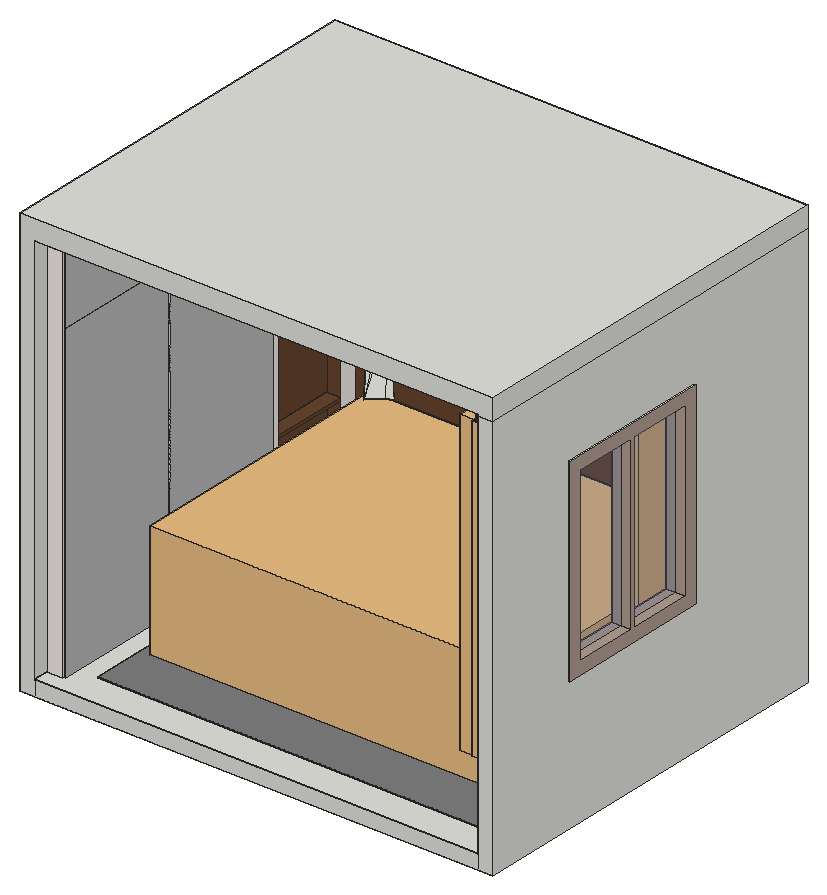
# SketchUp Ruby script. Lengths in inches.
U = 1.inch
M = Sketchup.active_model
def pt(a) = Geom::Point3d.new(a.map { |v| v * U })
def face(e, loops, mat)
  f = e.add_face(loops[0].map { |a| pt(a) })
  loops[1..].each { |l| e.add_face(l.map { |a| pt(a) }).erase! }
  f.material = f.back_material = mat if mat
  f
end
# faces: each face lists its corners as indices into pts; further lists are holes
def faces(e, pts, list, mat = nil) = list.each { |f| face(e, (f[0].is_a?(Array) ? f : [f]).map { |l| l.map { |i| pts[i] } }, mat) }
# xy, xz, yz: faces in a plane at the given z, y or x. An outline is a flat list of corners, or four numbers for a rectangle; further outlines are holes
def ring(l) = l.size == 4 ? [[l[0], l[1]], [l[2], l[1]], [l[2], l[3]], [l[0], l[3]]] : l.each_slice(2).to_a
def flat(e, list, mat, &to3) = list.each { |f| face(e, (f[0].is_a?(Array) ? f : [f]).map { |l| ring(l).map { |u, v| to3.(u, v) } }, mat) }
def xy(e, z, list, mat = nil) = flat(e, list, mat) { |x, y| [x, y, z] }
def xz(e, y, list, mat = nil) = flat(e, list, mat) { |x, z| [x, y, z] }
def yz(e, x, list, mat = nil) = flat(e, list, mat) { |y, z| [x, y, z] }
def lines(e, pts, list) = list.each { |a, b| e.add_line(pt(pts[a]), pt(pts[b])) }
# prism: a flat outline (further loops are holes) pulled along v
def prism(e, loops, v, mat = nil)
  f = face(e, loops, mat); d = Geom::Vector3d.new(v.map { |x| x * U })
  f.pushpull(f.normal.samedirection?(d) ? d.length : -d.length)
end
def box(e, o, s, mat = nil) = prism(e, [[o, [o[0] + s[0], o[1], o[2]], [o[0] + s[0], o[1] + s[1], o[2]], [o[0], o[1] + s[1], o[2]]]], [0, 0, s[2]], mat)
def at(x, y, z, deg = 0) = Geom::Transformation.translation(pt([x, y, z])) * Geom::Transformation.rotation(ORIGIN, Z_AXIS, deg.degrees)
def axes(o, x, y, z) = Geom::Transformation.new([*x, 0, *y, 0, *z, 0, *pt(o).to_a, 1])
def part(name) = M.definitions.add(name)
# library, detail: a bought-in or finely detailed component or shape, given as its bounding box
def library(name, o, s) = part(name).tap { |d| box(d.entities, o, s) }
def detail(e, o, s) = box(e.add_group.entities, o, s)
def put(e, d, t, mat = nil) = e.add_instance(d, t).tap { |i| i.material = mat if mat }
def group(e, t, mat = nil) = e.add_group.tap { |g| g.transformation = t; g.material = mat if mat }.entities
root = M.entities
M.materials.add("0209 AP 9428 SKY PINK").color = [243, 236, 233]
M.materials.add("2036 AP 8776 DARK ASH").color = [176, 158, 145]
M.materials.add("DDR840RVS01100X").color = [126, 127, 125]
M.materials.add("Glass_Mirror_01").color = [185, 185, 185]
M.materials.add("Glass_Sky Reflection_01").color = [126, 138, 183]
M.materials["Glass_Sky Reflection_01"].alpha = 0.25
M.materials.add("Wood_Veneer_15_1K").color = [103, 69, 45]
c1 = library("Double bed",[0,0,0],[83.59,112.46,35.43])
c2 = part("Carpet v15 (4)")
xy(c2.entities,0,[[-70.87,0,47.24,78.74]])
xy(c2.entities,0.39,[[-70.87,0,47.24,78.74]],"DDR840RVS01100X")
xz(c2.entities,0,[[-70.87,0,47.24,0.39]])
xz(c2.entities,78.74,[[-70.87,0,47.24,0.39]])
yz(c2.entities,-70.87,[[0,0,78.74,0.39]])
yz(c2.entities,47.24,[[0,0,78.74,0.39]])
c3 = part("Group\#8")
g1 = group(c3.entities,at(1.62,23.48,0.37))
prism(g1,[[[2.19,-1.21,0],[0.78,-1.47,0],[-0.07,3.1,0],[1.34,3.36,0]]],[0,0,0.04])
g2 = group(c3.entities,at(0,0,0))
xy(g2,0.33,[[3.33,0,0,23.09,1.89,23.4375],[3.33,0,1.89,23.4375,2.83,23.62],[3.33,0,2.83,23.62,4.25,23.88,8.53,0.97,7.12,0.71]])
xy(g2,0.37,[[3.33,0,1.89,23.4375,0,23.09],[3.33,0,2.83,23.62,1.89,23.4375],[3.33,0,7.12,0.71,8.53,0.97,4.25,23.88,2.83,23.62]])
p = [[5.64,24.14,0.12],[4.25,23.88,0.37],[8.53,0.97,0.37],[10.39,1.32,0.04],[4.25,23.88,0.33],[5.64,24.14,0.08],
  [10.39,1.32,0],[8.53,0.97,0.33],[2.83,23.62,0.33],[1.89,23.4375,0.33],[0,23.09,0.33],[0,23.09,0.37],
  [1.89,23.4375,0.37],[2.83,23.62,0.37],[3.33,0,0.33],[3.33,0,0.37],[7.12,0.71,0.37],[7.12,0.71,0.33]]
faces(g2,p,[[0,1,2,3],[4,5,6,7],[6,3,2,7],[5,0,3,6],[0,5,4,8,9,10,11,12,13,1],[14,15,11,10],[7,2,16,15,14,17]])
c4 = part("ceiling fan")
g3 = group(c4.entities,at(0.63,30.3,-2.8,-91.2))
g4 = group(g3,at(24.19,24.96,0))
xy(g4,0,[[4.53,2.58,4.03,2.65,3.56,2.84,3.16,3.15,2.85,3.55,2.65,4.02,2.58,4.52,2.65,5.02,2.84,5.5,3.15,5.9,3.55,6.21,4.02,6.41,4.52,6.47,5.02,6.41,5.5,6.22,5.9,5.91,6.21,5.51,6.41,5.04,6.47,4.53,6.41,4.03,6.22,3.56,5.91,3.16,5.51,2.85,5.04,2.65]])
xy(g4,2.76,[[4.54,0,5.71,0.16,6.8,0.61,7.74,1.34,8.46,2.28,8.9,3.37,9.06,4.54,8.9,5.71,8.44,6.8,7.72,7.74,6.78,8.46,5.68,8.9,4.51,9.06,3.34,8.9,2.25,8.44,1.32,7.72,0.6,6.78,0.15,5.68,0,4.51,0.16,3.34,0.61,2.25,1.34,1.32,2.28,0.6,3.37,0.15]])
p = [[4.54,0,1.57],[3.37,0.15,1.57],[4.03,2.65,0],[4.53,2.58,0],[5.71,0.16,1.57],[5.04,2.65,0],
  [2.28,0.6,1.57],[3.56,2.84,0],[6.8,0.61,1.57],[5.51,2.85,0],[1.34,1.32,1.57],[3.16,3.15,0],
  [7.74,1.34,1.57],[5.91,3.16,0],[0.61,2.25,1.57],[2.85,3.55,0],[8.46,2.28,1.57],[6.22,3.56,0],
  [0.16,3.34,1.57],[2.65,4.02,0],[8.9,3.37,1.57],[6.41,4.03,0],[0,4.51,1.57],[2.58,4.52,0],
  [9.06,4.54,1.57],[6.47,4.53,0],[0.15,5.68,1.57],[2.65,5.02,0],[8.9,5.71,1.57],[6.41,5.04,0],
  [0.6,6.78,1.57],[2.84,5.5,0],[8.44,6.8,1.57],[6.21,5.51,0],[1.32,7.72,1.57],[3.15,5.9,0],
  [7.72,7.74,1.57],[5.9,5.91,0],[2.25,8.44,1.57],[3.55,6.21,0],[6.78,8.46,1.57],[5.5,6.22,0],
  [3.34,8.9,1.57],[4.02,6.41,0],[5.68,8.9,1.57],[5.02,6.41,0],[4.51,9.06,1.57],[4.52,6.47,0],
  [3.37,0.15,2.76],[4.54,0,2.76],[5.71,0.16,2.76],[2.28,0.6,2.76],[6.8,0.61,2.76],[1.34,1.32,2.76],
  [7.74,1.34,2.76],[0.61,2.25,2.76],[8.46,2.28,2.76],[0.16,3.34,2.76],[8.9,3.37,2.76],[0,4.51,2.76],
  [9.06,4.54,2.76],[0.15,5.68,2.76],[8.9,5.71,2.76],[0.6,6.78,2.76],[8.44,6.8,2.76],[1.32,7.72,2.76],
  [7.72,7.74,2.76],[2.25,8.44,2.76],[6.78,8.46,2.76],[3.34,8.9,2.76],[5.68,8.9,2.76],[4.51,9.06,2.76]]
faces(g4,p,[[0,1,2,3],[4,0,3,5],[1,6,7,2],[8,4,5,9],[6,10,11,7],[12,8,9,13],[10,14,15,11],[16,12,13,17],
  [14,18,19,15],[20,16,17,21],[18,22,23,19],[24,20,21,25],[22,26,27,23],[28,24,25,29],[26,30,31,27],[32,28,29,33],
  [30,34,35,31],[36,32,33,37],[34,38,39,35],[40,36,37,41],[38,42,43,39],[44,40,41,45],[42,46,47,43],[46,44,45,47],
  [48,1,0,49],[49,0,4,50],[51,6,1,48],[50,4,8,52],[53,10,6,51],[52,8,12,54],[55,14,10,53],[54,12,16,56],
  [57,18,14,55],[56,16,20,58],[59,22,18,57],[58,20,24,60],[61,26,22,59],[60,24,28,62],[63,30,26,61],[62,28,32,64],
  [65,34,30,63],[64,32,36,66],[67,38,34,65],[66,36,40,68],[69,42,38,67],[68,40,44,70],[71,46,42,69],[70,44,46,71]])
put(g3,c3,at(26.98,0,2.42))
put(g3,c3,at(4.05,45.73,2.42,-120))
put(g3,c3,at(55.12,42.72,2.42,120))
g5 = group(g3,at(25.76,26.53,17.72))
p = [[2.95,2.95,7.28],[2.95,2.95,5.91]]
lines(g5,p,[[0,1]])
g6 = group(g5,at(0,0,5.91))
xy(g6,-5.91,[[[2.95,1.99,2.7,2.02,2.47,2.12,2.27,2.27,2.12,2.47,2.02,2.7,1.99,2.95,2.02,3.2,2.12,3.4375,2.27,3.64,2.47,3.79,2.7,3.89,2.95,3.92,3.2,3.89,3.4375,3.79,3.64,3.64,3.79,3.4375,3.89,3.2,3.92,2.95,3.89,2.7,3.79,2.47,3.64,2.27,3.4375,2.12,3.2,2.02],[2.95,2.38,3.1,2.4,3.24,2.46,3.36,2.55,3.45,2.67,3.5,2.81,3.52,2.95,3.5,3.1,3.45,3.24,3.36,3.36,3.24,3.45,3.1,3.5,2.95,3.52,2.81,3.5,2.67,3.45,2.55,3.36,2.46,3.24,2.4,3.1,2.38,2.95,2.4,2.81,2.46,2.67,2.55,2.55,2.67,2.46,2.81,2.4]]])
xy(g6,0,[[2.95,0,3.72,0.1,4.43,0.4,5.04,0.86,5.51,1.48,5.8,2.1875,5.91,2.95,5.8,3.72,5.51,4.43,5.04,5.04,4.43,5.51,3.72,5.8,2.95,5.91,2.1875,5.8,1.48,5.51,0.86,5.04,0.4,4.43,0.1,3.72,0,2.95,0.1,2.1875,0.4,1.48,0.86,0.86,1.48,0.4,2.1875,0.1]])
p = [[2.95,0,0],[2.1875,0.1,0],[2.7,2.02,-5.91],[2.95,1.99,-5.91],[3.72,0.1,0],[3.2,2.02,-5.91],
  [1.48,0.4,0],[2.47,2.12,-5.91],[4.43,0.4,0],[3.4375,2.12,-5.91],[0.86,0.86,0],[2.27,2.27,-5.91],
  [5.04,0.86,0],[3.64,2.27,-5.91],[0.4,1.48,0],[2.12,2.47,-5.91],[5.51,1.48,0],[3.79,2.47,-5.91],
  [0.1,2.1875,0],[2.02,2.7,-5.91],[5.8,2.1875,0],[3.89,2.7,-5.91],[0,2.95,0],[1.99,2.95,-5.91],
  [5.91,2.95,0],[3.92,2.95,-5.91],[0.1,3.72,0],[2.02,3.2,-5.91],[5.8,3.72,0],[3.89,3.2,-5.91],
  [0.4,4.43,0],[2.12,3.4375,-5.91],[5.51,4.43,0],[3.79,3.4375,-5.91],[0.86,5.04,0],[2.27,3.64,-5.91],
  [5.04,5.04,0],[3.64,3.64,-5.91],[1.48,5.51,0],[2.47,3.79,-5.91],[4.43,5.51,0],[3.4375,3.79,-5.91],
  [2.1875,5.8,0],[2.7,3.89,-5.91],[3.72,5.8,0],[3.2,3.89,-5.91],[2.95,5.91,0],[2.95,3.92,-5.91]]
faces(g6,p,[[0,1,2,3],[4,0,3,5],[1,6,7,2],[8,4,5,9],[6,10,11,7],[12,8,9,13],[10,14,15,11],[16,12,13,17],
  [14,18,19,15],[20,16,17,21],[18,22,23,19],[24,20,21,25],[22,26,27,23],[28,24,25,29],[26,30,31,27],[32,28,29,33],
  [30,34,35,31],[36,32,33,37],[34,38,39,35],[40,36,37,41],[38,42,43,39],[44,40,41,45],[42,46,47,43],[46,44,45,47]])
g7 = group(g3,at(25.76,26.53,1.46))
xy(g7,0,[[2.95,0,3.72,0.1,4.43,0.4,5.04,0.86,5.51,1.48,5.8,2.1875,5.91,2.95,5.8,3.72,5.51,4.43,5.04,5.04,4.43,5.51,3.72,5.8,2.95,5.91,2.1875,5.8,1.48,5.51,0.86,5.04,0.4,4.43,0.1,3.72,0,2.95,0.1,2.1875,0.4,1.48,0.86,0.86,1.48,0.4,2.1875,0.1]])
xy(g7,5.91,[[[2.95,1.99,2.7,2.02,2.47,2.12,2.27,2.27,2.12,2.47,2.02,2.7,1.99,2.95,2.02,3.2,2.12,3.4375,2.27,3.64,2.47,3.79,2.7,3.89,2.95,3.92,3.2,3.89,3.4375,3.79,3.64,3.64,3.79,3.4375,3.89,3.2,3.92,2.95,3.89,2.7,3.79,2.47,3.64,2.27,3.4375,2.12,3.2,2.02],[2.95,2.38,3.1,2.4,3.24,2.46,3.36,2.55,3.45,2.67,3.5,2.81,3.52,2.95,3.5,3.1,3.45,3.24,3.36,3.36,3.24,3.45,3.1,3.5,2.95,3.52,2.81,3.5,2.67,3.45,2.55,3.36,2.46,3.24,2.4,3.1,2.38,2.95,2.4,2.81,2.46,2.67,2.55,2.55,2.67,2.46,2.81,2.4]]])
p = [[2.95,0,0],[2.1875,0.1,0],[2.7,2.02,5.91],[2.95,1.99,5.91],[3.72,0.1,0],[3.2,2.02,5.91],
  [1.48,0.4,0],[2.47,2.12,5.91],[4.43,0.4,0],[3.4375,2.12,5.91],[0.86,0.86,0],[2.27,2.27,5.91],
  [5.04,0.86,0],[3.64,2.27,5.91],[0.4,1.48,0],[2.12,2.47,5.91],[5.51,1.48,0],[3.79,2.47,5.91],
  [0.1,2.1875,0],[2.02,2.7,5.91],[5.8,2.1875,0],[3.89,2.7,5.91],[0,2.95,0],[1.99,2.95,5.91],
  [5.91,2.95,0],[3.92,2.95,5.91],[0.1,3.72,0],[2.02,3.2,5.91],[5.8,3.72,0],[3.89,3.2,5.91],
  [0.4,4.43,0],[2.12,3.4375,5.91],[5.51,4.43,0],[3.79,3.4375,5.91],[0.86,5.04,0],[2.27,3.64,5.91],
  [5.04,5.04,0],[3.64,3.64,5.91],[1.48,5.51,0],[2.47,3.79,5.91],[4.43,5.51,0],[3.4375,3.79,5.91],
  [2.1875,5.8,0],[2.7,3.89,5.91],[3.72,5.8,0],[3.2,3.89,5.91],[2.95,5.91,0],[2.95,3.92,5.91]]
faces(g7,p,[[0,1,2,3],[4,0,3,5],[1,6,7,2],[8,4,5,9],[6,10,11,7],[12,8,9,13],[10,14,15,11],[16,12,13,17],
  [14,18,19,15],[20,16,17,21],[18,22,23,19],[24,20,21,25],[22,26,27,23],[28,24,25,29],[26,30,31,27],[32,28,29,33],
  [30,34,35,31],[36,32,33,37],[34,38,39,35],[40,36,37,41],[38,42,43,39],[44,40,41,45],[42,46,47,43],[46,44,45,47]])
g8 = group(g3,at(25.76,26.53,27.76))
prism(g8,[[[2.95,2.38,-20.39],[2.81,2.4,-20.39],[2.67,2.46,-20.39],[2.55,2.55,-20.39],[2.46,2.67,-20.39],[2.4,2.81,-20.39],[2.38,2.95,-20.39],[2.4,3.1,-20.39],[2.46,3.24,-20.39],[2.55,3.36,-20.39],[2.67,3.45,-20.39],[2.81,3.5,-20.39],[2.95,3.52,-20.39],[3.1,3.5,-20.39],[3.24,3.45,-20.39],[3.36,3.36,-20.39],[3.45,3.24,-20.39],[3.5,3.1,-20.39],[3.52,2.95,-20.39],[3.5,2.81,-20.39],[3.45,2.67,-20.39],[3.36,2.55,-20.39],[3.24,2.46,-20.39],[3.1,2.4,-20.39]]],[0,0,10.35])
c5 = part("Group28\#2")
xy(c5.entities,0,[[-20.0625,-26.0625,-0.59,26.0625],[0.59,-26.0625,20.0625,26.0625]])
c6 = library("Group16",[86.37,-10.76,76.46],[21.79,14.87,35.97])
c7 = library("Group22",[48.82,-10.91,0.23],[97.72,18.57,293.12])
c8 = library("Group24",[44.03,2.01,0.26],[103.73,11,292.35])
c9 = library("Group27",[-106.21,-10.76,76.46],[21.8,14.87,35.97])
c10 = library("Group35",[-145.81,2.01,0.26],[103.73,11,292.35])
c11 = library("Group33",[-144.59,-10.91,0.23],[97.72,18.57,293.12])
xy(root,-4.39,[[0,0,144,120]])
xy(root,0,[[4.5,0,139.5,0,139.5,115.5,9.5,115.5,9.5,110.5,5,110.5,5,86.5,9.5,86.5,9.5,4.5,4.5,4.5]])
xy(root,0.39,[[4.5,0,139.5,0,139.5,115.5,139.26,115.5,139.26,114.79,122.85,114.79,122.85,115.5,9.5,115.5,9.5,110.5,5,110.5,5,86.5,9.5,86.5,9.5,4.5,4.5,4.5],[135.32,102.33,139.5,109.79],[122.85,114.79,139.26,115.5]])
xy(root,0.63,[[9.5,4.74,10.21,44.06],[9.5,44.29,10.21,83.62]])
xy(root,29.61,[[5,86.5,9.5,110.5]],"Wood_Veneer_15_1K")
xy(root,30.39,[[5,86.5,9.5,110.5]],"Wood_Veneer_15_1K")
xy(root,36.39,[[139.5,28.5,141.75,76.5],[141.75,28.5,144,76.5],[144,28.5,144.6875,76.5]])
xy(root,36.39,[[138.8125,28.5,139.5,76.5]],"2036 AP 8776 DARK ASH")
xy(root,40.33,[[138.8125,32.4375,144.6875,51.91],[138.8125,53.09,144.6875,72.5625]],"2036 AP 8776 DARK ASH")
xy(root,48,[[122.85,114.79,139.26,115.5]])
xy(root,48.24,[[9.74,114.79,26.86,115.5],[27.1,114.79,45.19,115.5],[45.43,114.79,80.1,115.5],[80.34,114.79,106.69,115.5],[106.93,114.79,122.48,115.5],
  [122.71,114.79,139.26,115.5]])
xy(root,59.58,[[5,86.5,9.5,110.5]],"Wood_Veneer_15_1K")
xy(root,60.39,[[5,86.5,9.5,110.5]],"Wood_Veneer_15_1K")
xy(root,89.61,[[5,86.5,9.5,110.5]],"Wood_Veneer_15_1K")
xy(root,90.39,[[5,86.5,9.5,110.5]])
xy(root,92.46,[[138.8125,32.4375,144.6875,51.91],[138.8125,53.09,144.6875,72.5625]])
xy(root,95.83,[[9.5,4.74,10.21,44.06],[9.5,44.29,10.21,83.62]])
xy(root,96.07,[[9.5,4.74,10.21,44.06],[9.5,44.29,10.21,83.62]])
xy(root,96.39,[[139.5,28.5,141.75,76.5],[141.75,28.5,144,76.5],[144,28.5,144.6875,76.5]])
xy(root,96.39,[[138.8125,28.5,139.5,76.5]],"2036 AP 8776 DARK ASH")
xy(root,114.61,[[135.32,4.5,135.25,109.79,139.43,109.79,139.5,4.5]])
xy(root,119.37,[[9.5,4.74,10.21,44.06],[9.5,44.29,10.21,83.62]])
xy(root,119.61,[[9.74,114.79,26.86,115.5],[27.1,114.79,45.19,115.5],[45.43,114.79,80.1,115.5],[80.34,114.79,106.69,115.5],[106.93,114.79,122.48,115.5],
  [122.71,114.79,139.26,115.5]])
xy(root,120,[[[4.5,0,4.5,4.5,9.5,4.5,9.5,86.5,5,86.5,5,110.5,9.5,110.5,9.5,115.5,139.5,115.5,139.5,0],[25.7,16.2,123.3,99.3]],[135.32,4.5,139.5,4.5,139.43,109.79,135.25,109.79]])
xy(root,121.5,[[22.82,16.2,25.7,99.3],[123.3,16.2,126.18,102.18],[22.82,99.3,123.3,102.18]])
xy(root,123,[[22.82,16.2,126.18,102.18]])
xy(root,126,[[0,0,144,120]])
xz(root,0,[[0,-4.39,4.5,-4.39,4.5,120,139.5,120,139.5,119.61,144,119.61,144,126,0,126],[4.5,-4.39,139.5,0],[139.5,-4.39,144,119.61]])
xz(root,4.5,[[135.32,114.61,139.5,119.61],[4.5,119.61,9.5,120],[135.32,119.61,139.5,120],[4.5,120,9.5,120.39]])
xz(root,4.5,[[4.5,0.39,9.5,119.61]],"0209 AP 9428 SKY PINK")
xz(root,4.74,[[9.5,0.63,10.21,95.83],[9.5,96.07,10.21,119.37]])
xz(root,16.2,[[25.7,120,25.7,121.5,22.82,121.5,22.82,123,126.18,123,126.18,121.5,123.3,121.5,123.3,120]])
xz(root,28.5,[[139.5,36.39,141.75,96.39],[141.75,36.39,144,96.39],[144,36.39,144.6875,96.39]])
xz(root,28.5,[[138.8125,36.39,139.5,96.39]],"2036 AP 8776 DARK ASH")
xz(root,32.4375,[[138.8125,40.33,144.6875,92.46]])
xz(root,44.06,[[9.5,0.63,10.21,95.83],[9.5,96.07,10.21,119.37]])
xz(root,44.29,[[9.5,0.63,10.21,95.83],[9.5,96.07,10.21,119.37]])
xz(root,51.91,[[138.8125,40.33,144.6875,92.46]],"2036 AP 8776 DARK ASH")
xz(root,53.09,[[138.8125,40.33,144.6875,92.46]])
xz(root,72.5625,[[138.8125,40.33,144.6875,92.46]],"2036 AP 8776 DARK ASH")
xz(root,76.5,[[138.8125,36.39,139.5,96.39],[139.5,36.39,141.75,96.39],[141.75,36.39,144,96.39],[144,36.39,144.6875,96.39]])
xz(root,83.62,[[9.5,0.63,10.21,95.83],[9.5,96.07,10.21,119.37]])
xz(root,86.5,[[5,0,9.5,0.39],[5,0.39,9.5,29.61],[5,29.61,9.5,30],[5,30,9.5,30.39],[5,30.39,9.5,59.58],
  [5,60.39,9.5,89.61],[5,90.39,9.5,119.61],[5,119.61,9.5,120],[5,120,9.5,120.39]])
xz(root,99.3,[[25.7,120,123.3,121.5]])
xz(root,102.18,[[22.82,121.5,126.18,123]])
xz(root,102.33,[[135.32,0.39,139.5,0.39,139.43,114.61,135.25,114.6]],"0209 AP 9428 SKY PINK")
xz(root,109.79,[[135.32,0.39,135.25,114.6,139.43,114.61,139.5,0.39],[135.25,114.61,139.43,120]])
xz(root,110.5,[[5,29.61,9.5,30.39],[5,119.61,9.5,120],[5,120,9.5,120.39]])
xz(root,110.5,[[5,0.39,9.5,29.61],[5,30.39,9.5,59.58],[5,60.39,9.5,89.61],[5,90.39,9.5,119.61]],"Wood_Veneer_15_1K")
xz(root,114.79,[[9.74,48.24,26.86,119.61],[27.1,48.24,45.19,119.61],[45.43,48.24,80.1,119.61],[80.34,48.24,106.69,119.61],[106.93,48.24,122.48,119.61],
  [122.71,48.24,139.26,119.61]])
xz(root,114.79,[[122.85,0.39,139.26,48]],"0209 AP 9428 SKY PINK")
xz(root,115.5,[[122.61,0.39,122.85,48],[139.26,0.39,139.5,48],[[9.5,48,139.5,48,139.5,119.61,139.26,119.61,139.26,48.24,122.71,48.24,122.71,119.61,139.5,119.61,139.5,120,9.5,120,9.5,119.61,26.86,119.61,26.86,48.24,9.74,48.24,9.74,119.61,9.5,119.61],[45.43,48.24,80.1,119.61],[80.34,48.24,106.69,119.61],[27.1,48.24,45.19,119.61],[106.93,48.24,122.48,119.61]],[9.5,120,139.5,120.39]])
xz(root,115.5,[[9.5,0.39,122.61,48]],"Wood_Veneer_15_1K")
xz(root,120,[[0,-4.39,144,0],[0,0,144,0.39],[0,0.39,144,119.61],[0,119.61,144,120],[0,120,144,120.39],
  [0,120.39,144,126]])
yz(root,0,[[0,-4.39,120,0],[0,0,120,0.39],[0,0.39,120,120.39],[0,120.39,120,126]])
yz(root,4.5,[[0,0,4.5,0.39],[0,0.39,4.5,120]])
yz(root,5,[[86.5,29.61,110.5,30.39],[86.5,119.61,110.5,120],[86.5,120,110.5,120.39]])
yz(root,5,[[86.5,0.39,110.5,29.61],[86.5,30.39,110.5,59.58],[86.5,60.39,110.5,89.61],[86.5,90.39,110.5,119.61]],"Wood_Veneer_15_1K")
yz(root,9.5,[[[4.5,0.39,83.85,119.61],[4.74,0.63,44.06,119.37],[44.29,0.63,83.62,119.37]],[4.74,95.83,44.06,96.07],[44.29,95.83,83.62,96.07],[4.5,119.61,86.5,120],[110.5,119.61,115.5,120],
  [4.5,120,86.5,120.39],[110.5,120,115.5,120.39]])
yz(root,9.5,[[83.85,0.39,86.5,119.61],[110.5,0.39,115.5,119.61]],"0209 AP 9428 SKY PINK")
yz(root,9.5,[[86.5,29.61,110.5,30.39],[86.5,59.58,110.5,60.39],[86.5,89.61,110.5,90.39]],"Wood_Veneer_15_1K")
yz(root,9.74,[[114.79,48.24,115.5,119.61]])
yz(root,10.21,[[44.06,7.03,44.29,95.83]])
yz(root,10.21,[[4.74,0.63,44.06,95.83],[44.29,0.63,83.62,7.03],[44.29,7.03,83.62,95.83],[4.74,96.07,44.06,119.37],[44.29,96.07,83.62,119.37]],"Glass_Mirror_01")
yz(root,22.82,[[16.2,121.5,102.18,123]])
yz(root,25.7,[[16.2,120,99.3,121.5]])
yz(root,26.86,[[114.79,48.24,115.5,119.61]])
yz(root,27.1,[[114.79,48.24,115.5,119.61]])
yz(root,45.19,[[114.79,48.24,115.5,119.61]])
yz(root,45.43,[[114.79,48.24,115.5,119.61]])
yz(root,80.1,[[114.79,48.24,115.5,119.61]])
yz(root,80.34,[[114.79,48.24,115.5,119.61]])
yz(root,106.69,[[114.79,48.24,115.5,119.61]])
yz(root,106.93,[[114.79,48.24,115.5,119.61]])
yz(root,122.48,[[114.79,48.24,115.5,119.61]])
yz(root,122.71,[[114.79,48.24,115.5,119.61]])
yz(root,122.85,[[114.79,0.39,115.5,48]])
yz(root,123.3,[[16.2,120,99.3,121.5]])
yz(root,126.18,[[16.2,121.5,102.18,123]])
yz(root,138.8125,[[[28.5,36.39,76.5,96.39],[53.09,40.33,72.5625,92.46],[32.4375,40.33,51.91,92.46]]],"2036 AP 8776 DARK ASH")
yz(root,139.26,[[114.79,0.39,115.5,48],[114.79,48.24,115.5,119.61]])
yz(root,139.5,[[0,0,4.5,0.39],[4.5,0,115.5,0.39],[109.79,0.39,115.5,119.61,115.5,0.39],[4.5,114.61,4.5,119.61,115.5,119.61],[0,119.61,4.5,120],
  [4.5,119.61,115.5,120],[4.5,120,115.5,120.39]])
yz(root,139.5,[[0,0.39,4.5,119.61],[4.5,0.39,28.5,36.39,102.33,0.39],[4.5,0.39,28.5,96.39,28.5,36.39],[4.5,0.39,4.5,114.61,28.5,96.39],[102.33,0.39,28.5,36.39,76.5,36.39],
  [28.5,96.39,4.5,114.61,115.5,119.61]],"0209 AP 9428 SKY PINK")
yz(root,144,[[[0,-4.39,120,119.61],[28.5,36.39,76.5,96.39]],[0,119.61,120,126]])
yz(root,144.6875,[[[28.5,36.39,76.5,96.39],[53.09,40.33,72.5625,92.46],[32.4375,40.33,51.91,92.46]]],"2036 AP 8776 DARK ASH")
p = [[139.43,102.33,114.61],[139.5,102.33,0.39],[139.5,76.5,36.39],[135.32,109.79,0.39],[135.32,102.33,0.39],[135.25,102.33,114.6],
  [135.25,109.79,114.6],[139.5,109.79,0.39],[139.43,109.79,114.61],[139.5,115.5,119.61],[139.5,76.5,96.39],[139.5,28.5,96.39],
  [135.32,4.5,120],[135.25,109.79,120],[135.25,109.79,114.61],[135.32,4.5,114.61],[135.32,4.5,119.61],[139.43,109.79,120],
  [139.5,4.5,120],[139.5,4.5,119.61],[139.5,4.5,114.61],[9.5,115.5,48],[4.5,115.5,48],[4.5,115.5,120],
  [139.5,4.5,120.39],[139.5,0,120.39],[139.5,115.5,-0.39],[139.5,115.5,0],[9.5,4.5,-0.39],[9.5,4.5,0],
  [9.5,86.5,-0.39],[9.5,86.5,0],[9.5,110.5,0.39],[9.5,110.5,0],[123.3,16.2,121.5],[123.3,14.89,121.5],
  [25.7,16.2,121.5],[25.7,8.19,121.5]]
faces(root,p,[[0,1,2],[3,4,5,6],[2,10,0],[0,11,9],[10,11,0]],"0209 AP 9428 SKY PINK")
faces(root,p,[[7,8,9],[12,13,14,15,16],[17,18,19,20,8],[0,8,6,5],[8,0,9]])
lines(root,p,[[21,22],[22,23],[24,25],[26,27],[28,29],[30,31],[32,33],[34,35],[36,37]])
put(root,c1,at(131.3,25.93,0.39,90))
put(root,c2,at(86.81,9.66,0.39))
put(root,c4,at(45.43,41.75,99.17))
put(root,c5,axes([141.75,52.5,66.39],[0,-1,0],[0,0,1],[-1,0,0]),"Glass_Sky Reflection_01")
put(root,c6,axes([129.32,50.7,22.875],[0,-0.3127,0],[0.3127,0,0],[0,0,0.3127]))
put(root,c7,axes([133.51,50.71,22.875],[0,-0.3127,0],[0.3127,0,0],[0,0,0.3127]))
put(root,c8,axes([133.51,50.71,22.875],[0,-0.3127,0],[0.3127,0,0],[0,0,0.3127]))
put(root,c9,axes([129.32,50.7,22.875],[0,-0.3127,0],[0.3127,0,0],[0,0,0.3127]))
put(root,c10,axes([133.51,50.71,22.875],[0,-0.3127,0],[0.3127,0,0],[0,0,0.3127]))
put(root,c11,axes([133.51,50.71,22.875],[0,-0.3127,0],[0.3127,0,0],[0,0,0.3127]))
